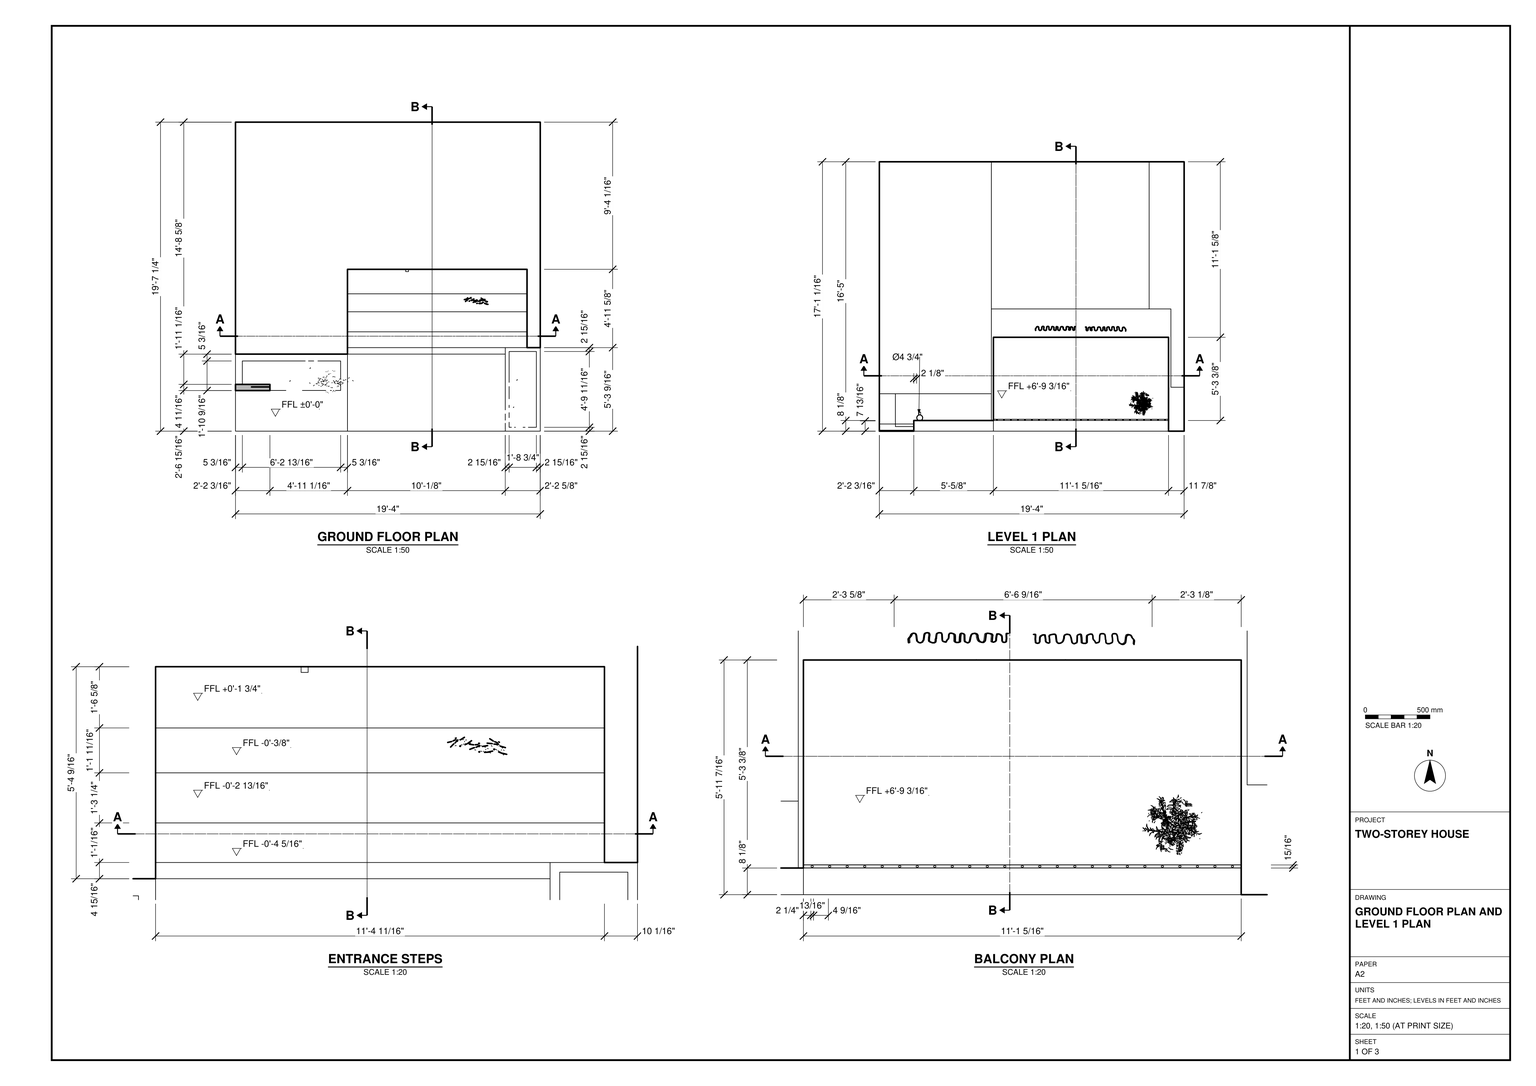
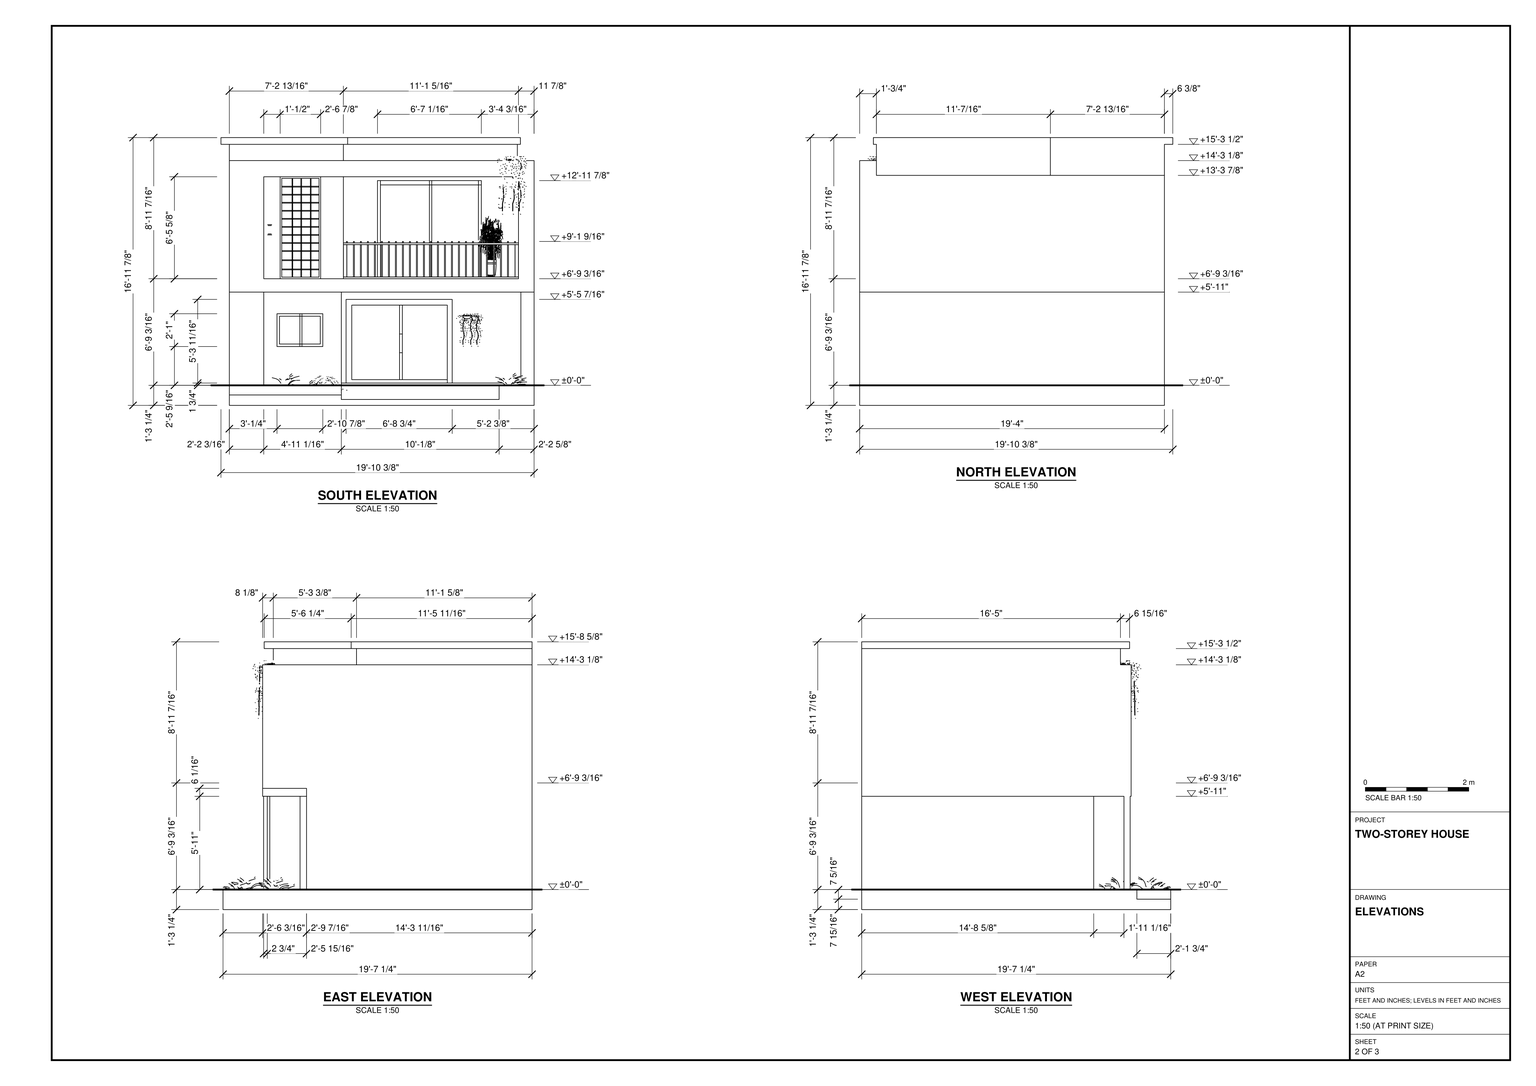
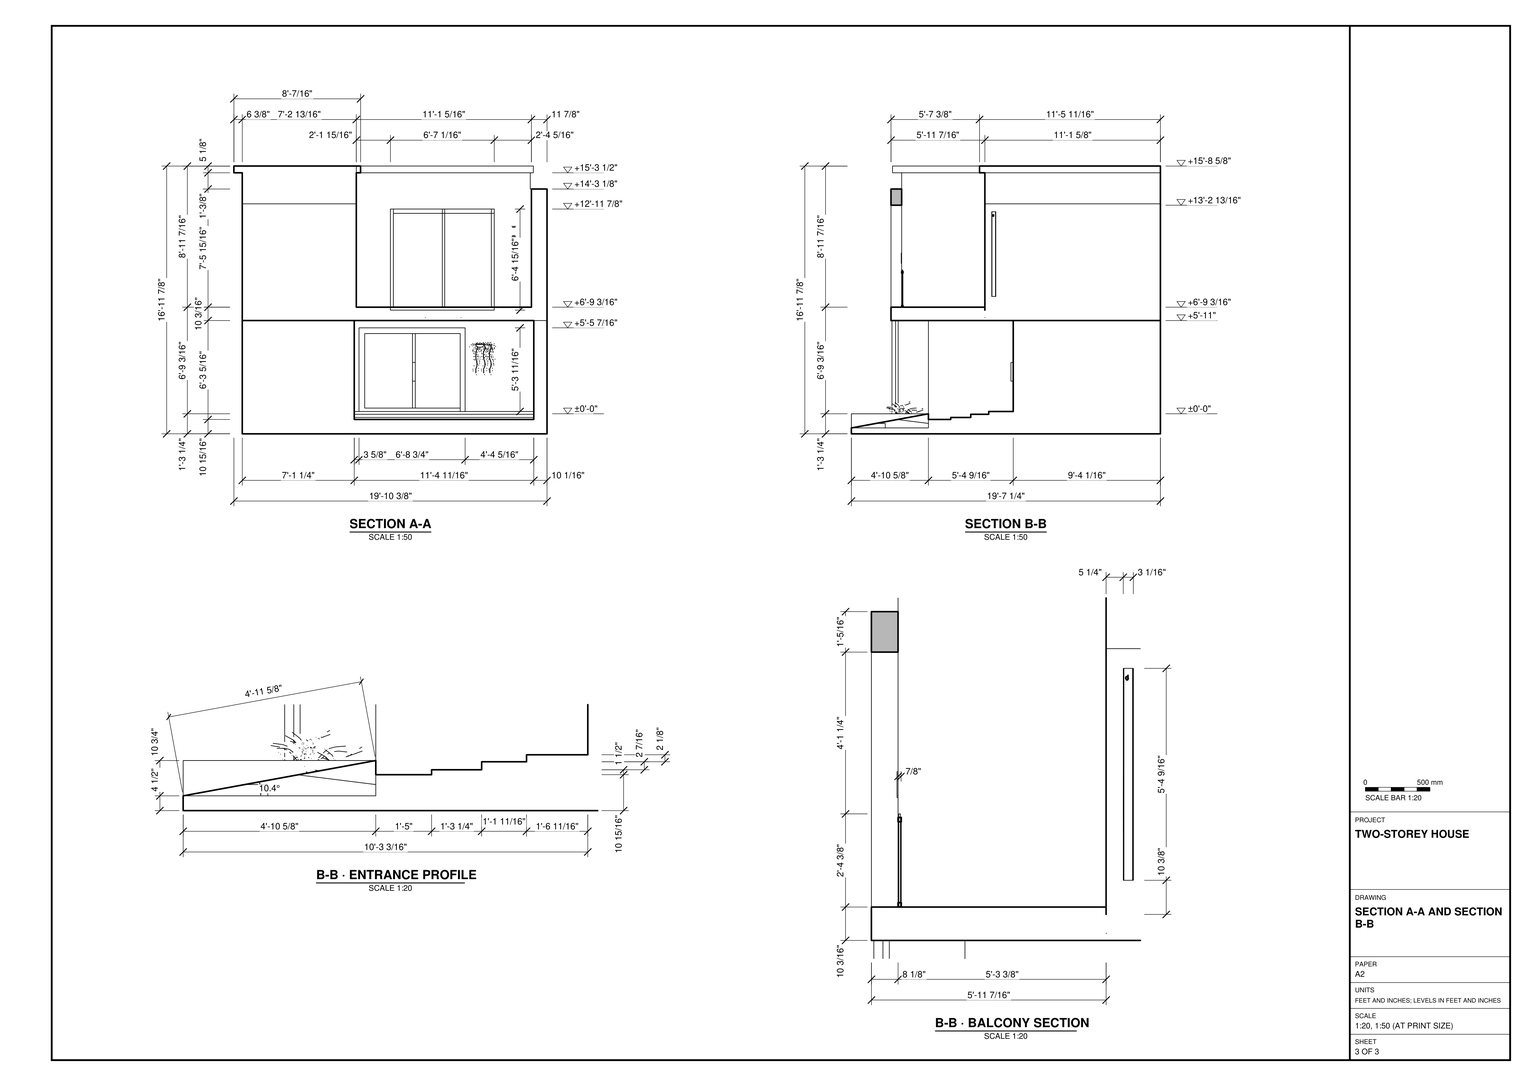
Work in feet and inches to model the two-storey house shown in task_files/diagram_01.pdf. The overall dimensions are 19'-10 3/8" along the south elevation, 19'-7 1/4" from front to back and 16'-11 7/8" high. Set the ground-floor level at ±0'-0" and the upper-floor level at +6'-9 3/16".

Build the base, exterior walls, floor slabs and flat roof with the thicknesses and setbacks shown in the plans and sections. Use the entrance profile on sheet 3 to shape the sloping approach and the shallow steps leading back to the recessed ground-floor entrance. On the south elevation, place the small divided window to the left of the wide glazed entrance. Above it, distinguish the tall gridded opening on the left from the paired glazed opening behind the balcony. Match the balcony footprint to its enlarged plan and place the railing along its outer edge. Include the planting at the entrance and balcony in the positions shown. Decor and loose items, including plants, may be any suitable library components.

Keep the walls, slabs and roof as separate groups or components. Keep each furniture or joinery piece separate and use components for repeated parts. Save one SketchUp model as output_files/two_storey_house_with_a_balcony_and_stepped_entrance.skp.

# SketchUp Ruby script. Lengths in inches.
U = 1.inch
M = Sketchup.active_model
def pt(a) = Geom::Point3d.new(a.map { |v| v * U })
def face(e, loops, mat)
  f = e.add_face(loops[0].map { |a| pt(a) })
  loops[1..].each { |l| e.add_face(l.map { |a| pt(a) }).erase! }
  f.material = f.back_material = mat if mat
  f
end
# faces: each face lists its corners as indices into pts; further lists are holes
def faces(e, pts, list, mat = nil) = list.each { |f| face(e, (f[0].is_a?(Array) ? f : [f]).map { |l| l.map { |i| pts[i] } }, mat) }
# xy, xz, yz: faces in a plane at the given z, y or x. An outline is a flat list of corners, or four numbers for a rectangle; further outlines are holes
def ring(l) = l.size == 4 ? [[l[0], l[1]], [l[2], l[1]], [l[2], l[3]], [l[0], l[3]]] : l.each_slice(2).to_a
def flat(e, list, mat, &to3) = list.each { |f| face(e, (f[0].is_a?(Array) ? f : [f]).map { |l| ring(l).map { |u, v| to3.(u, v) } }, mat) }
def xy(e, z, list, mat = nil) = flat(e, list, mat) { |x, y| [x, y, z] }
def xz(e, y, list, mat = nil) = flat(e, list, mat) { |x, z| [x, y, z] }
def yz(e, x, list, mat = nil) = flat(e, list, mat) { |y, z| [x, y, z] }
def lines(e, pts, list) = list.each { |a, b| e.add_line(pt(pts[a]), pt(pts[b])) }
# prism: a flat outline (further loops are holes) pulled along v
def prism(e, loops, v, mat = nil)
  f = face(e, loops, mat); d = Geom::Vector3d.new(v.map { |x| x * U })
  f.pushpull(f.normal.samedirection?(d) ? d.length : -d.length)
end
def box(e, o, s, mat = nil) = prism(e, [[o, [o[0] + s[0], o[1], o[2]], [o[0] + s[0], o[1] + s[1], o[2]], [o[0], o[1] + s[1], o[2]]]], [0, 0, s[2]], mat)
def at(x, y, z, deg = 0) = Geom::Transformation.translation(pt([x, y, z])) * Geom::Transformation.rotation(ORIGIN, Z_AXIS, deg.degrees)
def axes(o, x, y, z) = Geom::Transformation.new([*x, 0, *y, 0, *z, 0, *pt(o).to_a, 1])
def part(name) = M.definitions.add(name)
# library, detail: a bought-in or finely detailed component or shape, given as its bounding box
def library(name, o, s) = part(name).tap { |d| box(d.entities, o, s) }
def detail(e, o, s) = box(e.add_group.entities, o, s)
def put(e, d, t, mat = nil) = e.add_instance(d, t).tap { |i| i.material = mat if mat }
def group(e, t, mat = nil) = e.add_group.tap { |g| g.transformation = t; g.material = mat if mat }.entities
root = M.entities
M.materials.add("Leaf_Half_Top_007").color = [114, 127, 96]
M.materials.add("Niraj_Hair_Gray").color = [178, 178, 178]
M.materials.add("[Asphalt New]").color = [67, 60, 62]
M.materials.add("[Asphalt_New]").color = [58, 58, 58]
M.materials.add("[Color M08]").color = [30, 30, 30]
M.materials.add("[Color_F18]").color = [71, 102, 40]
M.materials.add("[Groundcover_Wood_Mix]").color = [22, 20, 19]
M.materials.add("[Metal Seamed]").color = [118, 119, 115]
M.materials.add("[Translucent Glass Gray]").color = [128, 128, 128]
M.materials["[Translucent Glass Gray]"].alpha = 0.5
M.materials.add("[Wood Board Cork]").color = [215, 201, 115]
c1 = part("Group\#428")
prism(c1.entities,[[[0,1.97,0],[0,1.97,1.18],[0,0,1.18],[0,0,0]],[[0,1.92,1.13],[0,1.92,0.05],[0,0.05,0.05],[0,0.05,1.13]]],[98.43,0,0])
c2 = part("Group\#430")
xy(c2.entities,0,[[0.3,0,0.22,0.01,0.15,0.04,0.09,0.09,0.04,0.15,0.01,0.22,0,0.3,0.3,0.3],[0.3,0,0.3,0.3,0.59,0.3,0.58,0.22,0.55,0.15,0.5,0.09,0.44,0.04,0.37,0.01],[0,0.3,0.01,0.37,0.04,0.44,0.09,0.5,0.15,0.55,0.22,0.58,0.3,0.59,0.3,0.3],[0.3,0.3,0.3,0.59,0.37,0.58,0.44,0.55,0.5,0.5,0.55,0.44,0.58,0.37,0.59,0.3]])
xy(c2.entities,39.37,[[0.3,0,0.37,0.01,0.44,0.04,0.5,0.09,0.55,0.15,0.58,0.22,0.59,0.3,0.58,0.37,0.55,0.44,0.5,0.5,0.44,0.55,0.37,0.58,0.3,0.59,0.22,0.58,0.15,0.55,0.09,0.5,0.04,0.44,0.01,0.37,0,0.3,0.01,0.22,0.04,0.15,0.09,0.09,0.15,0.04,0.22,0.01]])
p = [[0.09,0.09,0],[0.15,0.04,0],[0.15,0.04,39.37],[0.09,0.09,39.37],[0.22,0.01,0],[0.22,0.01,39.37],
  [0.3,0,0],[0.3,0,39.37],[0.37,0.01,0],[0.37,0.01,39.37],[0.44,0.04,0],[0.44,0.04,39.37],
  [0.5,0.09,0],[0.5,0.09,39.37],[0.01,0.22,0],[0.04,0.15,0],[0.04,0.15,39.37],[0.01,0.22,39.37],
  [0.55,0.15,0],[0.55,0.15,39.37],[0.58,0.22,0],[0.58,0.22,39.37],[0,0.3,0],[0,0.3,39.37],
  [0.59,0.3,0],[0.59,0.3,39.37],[0.01,0.37,0],[0.01,0.37,39.37],[0.58,0.37,0],[0.58,0.37,39.37],
  [0.09,0.5,0],[0.04,0.44,0],[0.04,0.44,39.37],[0.09,0.5,39.37],[0.55,0.44,0],[0.5,0.5,0],
  [0.5,0.5,39.37],[0.55,0.44,39.37],[0.15,0.55,0],[0.15,0.55,39.37],[0.44,0.55,0],[0.44,0.55,39.37],
  [0.22,0.58,0],[0.22,0.58,39.37],[0.3,0.59,0],[0.3,0.59,39.37],[0.37,0.58,0],[0.37,0.58,39.37]]
faces(c2.entities,p,[[0,1,2,3],[1,4,5,2],[4,6,7,5],[6,8,9,7],[8,10,11,9],[10,12,13,11],[14,15,16,17],[15,0,3,16],
  [12,18,19,13],[18,20,21,19],[22,14,17,23],[20,24,25,21],[26,22,23,27],[24,28,29,25],[30,31,32,33],[31,26,27,32],
  [34,35,36,37],[28,34,37,29],[38,30,33,39],[35,40,41,36],[42,38,39,43],[44,42,43,45],[46,44,45,47],[40,46,47,41]])
c3 = part("Group\#429")
prism(c3.entities,[[[0.01,0.22,35.83],[0,0.3,35.83],[0.01,0.37,35.83],[0.04,0.44,35.83],[0.09,0.5,35.83],[0.15,0.55,35.83],[0.22,0.58,35.83],[0.3,0.59,35.83],[0.37,0.58,35.83],[0.44,0.55,35.83],[0.5,0.5,35.83],[0.55,0.44,35.83],[0.58,0.37,35.83],[0.59,0.3,35.83],[0.58,0.22,35.83],[0.55,0.15,35.83],[0.5,0.09,35.83],[0.44,0.04,35.83],[0.37,0.01,35.83],[0.3,0,35.83],[0.22,0.01,35.83],[0.15,0.04,35.83],[0.09,0.09,35.83],[0.04,0.15,35.83]]],[0,0,3.54])
c4 = part("Metal railing panel")
g1 = group(c4.entities,at(0,0,0))
put(g1,c1,axes([0,0,39.76],[1,0,0],[0,0,-1],[0,1,0]),"[Color M08]")
put(g1,c1,axes([0,0,1.97],[1,0,0],[0,0,-1],[0,1,0]),"[Color M08]")
put(g1,c1,axes([98.43,0,37.8],[0,0,-0.364],[-1,0,0],[0,1,0]),"[Color M08]")
put(g1,c1,axes([1.97,0,37.8],[0,0,-0.364],[-1,0,0],[0,1,0]),"[Color M08]")
g2 = group(c4.entities,at(1.67,0.3,1.97))
put(g2,c2,at(78.74,0,0),"[Color M08]")
put(g2,c2,at(90.55,0,0),"[Color M08]")
put(g2,c2,at(82.68,0,0),"[Color M08]")
put(g2,c2,at(86.61,0,0),"[Color M08]")
put(g2,c2,at(66.93,0,0),"[Color M08]")
put(g2,c2,at(11.8125,0,0),"[Color M08]")
put(g2,c2,at(15.75,0,0),"[Color M08]")
put(g2,c2,at(47.24,0,0),"[Color M08]")
put(g2,c2,at(59.06,0,0),"[Color M08]")
put(g2,c3,at(0,0,0),"[Color M08]")
put(g2,c2,at(39.37,0,0),"[Color M08]")
put(g2,c2,at(62.99,0,0),"[Color M08]")
put(g2,c2,at(55.12,0,0),"[Color M08]")
put(g2,c2,at(19.69,0,0),"[Color M08]")
put(g2,c2,at(35.43,0,0),"[Color M08]")
put(g2,c2,at(7.875,0,0),"[Color M08]")
put(g2,c2,at(23.62,0,0),"[Color M08]")
put(g2,c2,at(31.5,0,0),"[Color M08]")
put(g2,c2,at(43.31,0,0),"[Color M08]")
put(g2,c2,at(27.56,0,0),"[Color M08]")
put(g2,c2,at(3.9375,0,0),"[Color M08]")
put(g2,c2,at(51.18,0,0),"[Color M08]")
put(g2,c2,at(70.87,0,0),"[Color M08]")
put(g2,c2,at(74.8,0,0),"[Color M08]")
put(g2,c3,at(94.49,0,0),"[Color M08]")
c5 = library("Broadleaf plant",[0,0,0],[149.19,166.1,98.1875])
c6 = library("TS_VASO+GANCHOS-PARA-PENDURAR\#1",[-17.61,-15.74,-70.29],[36.55,50.24,77.96])
c7 = part("Pot Half 03")
p = [[1.24,1.853,0],[6.161,1.853,0],[6.586,1.426,3.732],[0.815,1.426,3.732],[1.24,1.851,0],[6.161,7.34,0],
  [6.586,7.767,3.732],[6.679,1.345,4.342],[0.722,1.345,4.342],[6.679,7.848,4.342],[6.772,1.24,4.958],[0.629,1.24,4.958],
  [6.772,7.953,4.958],[6.906,1.118,5.538],[0.495,1.118,5.538],[6.906,8.075,5.538],[7.045,0.967,6.137],[0.356,0.967,6.137],
  [7.045,8.226,6.137],[7.221,0.804,6.691],[0.18,0.804,6.691],[7.221,8.389,6.691],[7.401,0.616,7.25],[0,0.616,7.25],
  [7.401,8.577,7.25]]
faces(c7.entities,p,[[0,1,2,3],[3,0,4],[5,6,2,1],[7,8,3,2],[9,7,2,6],[10,11,8,7],[12,10,7,9],[13,14,11,10],
  [15,13,10,12],[16,17,14,13],[18,16,13,15],[19,20,17,16],[21,19,16,18],[22,23,20,19],[24,22,19,21]],"[Asphalt_New]")
c8 = part("Dirt 003")
xy(c8.entities,-0.75,[[0,-3.72,3.43,-3.72,3.43,0],[-3.43,0,0,3.72,-3.43,3.72]])
p = [[-3.43,-3.72,-0.75],[0,0,0],[-3.43,0,-0.75],[0,-3.72,-0.75],[3.43,0,-0.75],[0,3.72,-0.75],
  [3.43,3.72,-0.75]]
faces(c8.entities,p,[[0,1,2],[0,3,1],[3,4,1],[2,1,5],[1,4,6],[1,6,5]])
c9 = part("Planter Box 01")
put(c9.entities,c7,axes([-30.22,-0.62,-6.86],[4.97512,0,0],[0,1,0],[0,0,1]),"[Asphalt_New]")
put(c9.entities,c7,axes([6.66,8.58,-6.86],[-4.97512,0,0],[0,-1,0],[0,0,1]))
put(c9.entities,c8,axes([-11.66,3.97,0.41],[4.97512,0,0],[0,1,0],[0,0,1]),"[Groundcover_Wood_Mix]")
c10 = part("Group8\#1")
p = [[88.35,32.45,7.18],[88.36,32.39,7.24],[86.45,32.02,7.22],[86.4375,32.08,7.17],[88.36,32.39,7.32],[86.45,32.02,7.3],
  [88.33,32.52,7.2],[86.42,32.16,7.1875],[88.32,32.56,7.28],[86.42,32.19,7.26],[90.24,33.16,7.22],[90.27,33.09,7.2],
  [90.29,33.02,7.26],[90.29,33.02,7.34],[90.23,33.19,7.3],[88.34,32.45,7.37],[86.4375,32.08,7.35],[88.32,32.52,7.35],
  [86.42,32.16,7.34],[90.27,33.08,7.39],[90.24,33.16,7.37]]
faces(c10.entities,p,[[0,1,2,3],[1,4,5,2],[6,0,3,7],[8,6,7,9],[10,11,0,6],[11,12,1,0],[12,13,4,1],[14,10,6,8],
  [4,15,16,5],[15,17,18,16],[17,8,9,18],[13,19,15,4],[19,20,17,15],[20,14,8,17]],"[Color_F18]")
c11 = part("Stem Segment 03")
put(c11.entities,c10,at(-88.34,-32.47,-7.28))
c12 = part("Leaf Stem 003")
p = [[2.85,0.02,0.06],[2.46,0.65,0.09],[2.46,0.65,0.03],[2.85,0.02,0.02],[2.92,0.03,0.01],[2.53,0.71,0.01],
  [2.55,0.72,0.0625],[2.93,0.04,0.04],[2.49,0.68,0],[2.89,0.01,0],[2.92,0.03,0.07],[2.53,0.71,0.11],
  [1.77,1.25,0.09],[1.77,1.25,0.03],[2.46,0.65,0.09],[1.8,1.29,0],[1.83,1.33,0.01],[1.84,1.35,0.0625],
  [1.38,1.49,0.09],[1.38,1.49,0.03],[1.43,1.57,0.01],[1.44,1.59,0.0625],[1.4,1.52,0],[0.375,2.11,0.09],
  [0.375,2.11,0.03],[0.39,2.15,0],[0.42,2.19,0.01],[0.43,2.22,0.0625],[0,2.29,0.05],[0.02,2.35,0],
  [0,2.29,0.13],[0,2.29,0.09],[0.04,2.43,0.02],[0.06,2.46,0.09],[2.49,0.68,0.12],[2.89,0.01,0.08],
  [1.83,1.33,0.11],[1.8,1.29,0.12],[1.4,1.52,0.12],[1.43,1.57,0.11],[0.42,2.19,0.11],[0.39,2.15,0.12],
  [0.02,2.35,0.1875],[0.04,2.43,0.17]]
faces(c12.entities,p,[[0,1,2,3],[4,5,6,7],[8,5,4,9],[10,7,6,11],[9,3,2,8],[12,13,2,14],[2,13,8],[15,8,13],
  [8,15,5],[16,5,15],[17,6,16],[5,16,6],[13,12,18,19],[17,16,20,21],[16,15,22,20],[15,13,19,22],
  [19,18,23,24],[22,19,24,25],[20,22,25,26],[21,20,26,27],[24,28,25],[29,25,28],[25,29,26],[30,31,28,24,23],
  [32,26,29],[33,27,32],[26,32,27],[34,35,10,11],[11,6,36],[17,36,6],[34,11,37],[36,37,11],
  [37,12,34],[14,34,12],[12,37,38,18],[37,36,39,38],[36,17,21,39],[38,39,40,41],[18,38,41,23],[39,21,27,40],
  [41,40,42],[30,23,41,42],[43,42,40],[40,27,43],[33,43,27]],"[Color_F18]")
c13 = part("Leaf stalk")
put(c13.entities,c12,at(0,0,0),"[Color_F18]")
c14 = part("Leaf Half 003\#2")
xz(c14.entities,0,[[5.394,0.387,3.719,3.029,4.031,3.19,4.352,3.332,4.681,3.455,5.017,3.558,5.359,3.64,5.704,3.702,6.053,3.743,6.404,3.763,6.755,3.762,6.968,3.765,7.18,3.761,7.392,3.75,7.604,3.731,7.815,3.706,8.025,3.674,8.234,3.635,8.442,3.589,8.648,3.537,8.852,3.478,9.054,3.412,9.254,3.339,9.523,3.226,9.776,3.081,10.009,2.905,10.218,2.701,10.4,2.473,10.553,2.224,10.674,1.959,10.76,1.68,10.803,1.439,10.807,1.344,10.806,1.249,10.8,1.154,10.788,1.059,10.772,0.965,10.749,0.873,10.722,0.781,10.689,0.69,10.652,0.602,10.609,0.515,10.562,0.43,10.535,0.387]],"Leaf_Half_Top_007")
p = [[0.878,-0.545,0.444],[0.896,-0.538,0.464],[0.931,-0.525,0.507],[0.966,-0.512,0.549],[1.39,-0.366,0.995],[1.791,-0.364,0.444],
  [2.095,-0.165,1.727],[1.842,-0.358,0.429],[1.796,-0.364,0.437],[2.997,-0.164,0.429],[2.858,-0.042,2.43],[3.012,-0.163,0.428],
  [4.203,-0.043,0.406],[2.861,-0.041,2.432],[3.719,0,3.029],[5.394,0,0.387],[2.302,-0.122,1.934],[2.485,-0.09,2.102],
  [2.671,-0.064,2.268],[3.132,-0.018,2.649],[3.418,-0.005,2.848]]
faces(c14.entities,p,[[0,1,2,3,4,5],[5,4,6,7,8],[7,6,9],[9,6,10,11],[11,10,12],[10,13,14,12],[15,12,14],[16,10,6],
  [17,10,16],[18,10,17],[19,14,13],[20,14,19]],"Leaf_Half_Top_007")
c15 = part("Leaf  003")
put(c15.entities,c14,axes([0.38,-0.76,0.25],[-0.73627,0.51406,-0.06038],[0.07956,0.22794,0.97042],[-0.56957,-0.78855,0.23191]))
put(c15.entities,c14,axes([-0.33,-1.74,0.14],[-0.71206,0.54726,-0.05889],[-0.2936,-0.28379,0.91283],[0.5365,0.74143,0.40305]))
c16 = part("Stem 03")
put(c16.entities,c11,axes([-3.94,-0.51,0],[1.00831,0.3173,0.48929],[0.62823,-0.33003,-1.08062],[-0.15419,1.18746,-0.4523]))
put(c16.entities,c11,axes([3.49,-0.02,-2.22],[0.59576,-0.02646,-0.80273],[0.76313,-0.29296,0.57602],[-0.25041,-0.95576,-0.15434]))
put(c16.entities,c11,axes([9.375,1.32,-6.76],[0.76506,0.42795,-0.48118],[0.54249,-0.02572,0.83967],[0.34696,-0.90343,-0.25184]))
put(c16.entities,c11,axes([6.35,0.02,-4.79],[0.59576,-0.02646,-0.80273],[0.35669,0.9042,0.23492],[0.71961,-0.42629,0.54812]))
put(c16.entities,c11,axes([12.62,2.51,-7.16],[0.6803,0.33788,-0.02508],[0.33232,-0.6545,0.19696],[0.06597,-0.18727,-0.73361]),"[Color_F18]")
put(c16.entities,c11,axes([0.3,0.04,-0.21],[-0.84454,-0.08139,0.52927],[-0.53545,0.11632,-0.83652],[0.00652,-0.98987,-0.14182]))
put(c16.entities,c13,axes([-1.3125,-1.96,2.02],[0.30666,0.85318,0.66121],[-0.04993,0.77839,-0.74104],[-2.0519,0.10857,0.11685]))
put(c16.entities,c13,axes([-4.65,-2.32,1.92],[0.24338,0.85318,0.71076],[0.37608,0.73871,-0.80238],[-1.59205,0.25393,-0.07463]))
put(c16.entities,c13,axes([-7.2,-3.29,1.22],[0.30238,0.83595,0.58629],[0.37608,0.73871,-0.65859],[-1.58433,0.30016,-0.01484]))
put(c16.entities,c13,axes([0.53,-1.96,0.51],[0.32572,0.6177,0.78674],[-0.09946,0.84405,-0.28154],[-1.60731,-0.00658,0.27494]))
put(c16.entities,c13,axes([3.92,-1.49,-0.93],[0.30617,0.58064,0.73954],[-0.72502,0.69723,-0.01619],[-1.09889,-0.4139,0.62826]))
put(c16.entities,c13,axes([4.9375,-1.13,-0.64],[0.15705,0.93505,0.23221],[-0.515,0.47073,-0.69124],[-1.33185,0.0406,0.34107]))
put(c16.entities,c13,axes([6.62,-2.02,-3.44],[0.25326,0.61577,0.6588],[-0.59973,0.73941,-0.01442],[-0.90899,-0.43895,0.55966]))
put(c16.entities,c13,axes([7.8,1.95,-4.46],[0.47026,-0.74247,0.15265],[-0.05932,-0.60353,-0.69183],[0.55983,0.33909,-0.83034]))
put(c16.entities,c13,axes([8.1,0.54,-5.54],[0.44324,0.59809,0.36462],[0.53568,0.30234,-0.47352],[-0.95326,0.41061,-0.31748]))
put(c16.entities,c13,axes([9.91,3.23,-5.95],[0.66281,-0.36564,0.35664],[0.55741,-0.47264,-0.48381],[0.53295,0.52862,-0.61482]))
put(c16.entities,c13,axes([13.4375,2.48,-5.88],[0.62226,-0.02903,-0.01582],[0.2868,0.07076,-0.50026],[-0.12016,0.85017,-0.2373]))
put(c16.entities,c15,axes([14.48,0.92,-5.23],[0.0087,-0.21722,0.04751],[0.21837,-0.00716,-0.09125],[0.14863,0.04515,0.19139]))
put(c16.entities,c15,axes([9.9,3.39,-4.35],[-0.29123,0.01957,0.06847],[-0.02535,-0.26587,-0.00841],[0.07568,-0.01372,0.26066]))
put(c16.entities,c15,axes([7.01,1.24,-3.35],[-0.21895,-0.20956,0.10962],[0.2232,-0.10618,-0.07961],[0.2062,0.0234,0.22464]))
put(c16.entities,c15,axes([9.1,-1.16,-2.97],[0.16646,-0.16408,0.06345],[0.32123,-0.02918,-0.16141],[0.19487,0.1494,0.19131]))
put(c16.entities,c15,axes([7.62,1.91,-0.74],[-0.13636,0.15771,0.21131],[-0.30082,-0.24908,0.19555],[0.22388,-0.05253,0.25505]))
put(c16.entities,c15,axes([6.63,0.34,1.27],[0.28289,-0.14866,0.08879],[0.17621,0.08243,-0.1563],[0.15509,0.20742,0.13835]))
put(c16.entities,c15,axes([5.87,-2.37,2.55],[0.24481,-0.24553,0.03382],[0.13933,0.2091,-0.24174],[0.19372,0.29074,0.28289]))
put(c16.entities,c15,axes([2.0625,1.79,5.35],[-0.18104,0.18123,0.28972],[-0.43052,-0.16317,-0.07437],[0.10324,-0.22668,0.29612]))
put(c16.entities,c15,axes([1.29,-0.99,6.37],[0.35078,-0.04064,0.25637],[0.22081,0.3154,-0.13622],[-0.24663,0.21043,0.25293]))
put(c16.entities,c13,axes([-3.94,-4.26,-2.18],[0.2039,-0.7121,1.03293],[-0.70199,1.01563,0.56503],[-1.36054,-0.65537,-0.37049]))
c17 = part("3D Plant 003")
put(c17.entities,c9,axes([2.34,-3.97,-0.41],[0.201,0,0],[0,1,0],[0,0,1]))
put(c17.entities,c16,axes([5.43,0.67,0.04],[0.90233,-0.11399,0],[0.12659,1.00204,0],[0,0,1]))
put(c17.entities,c16,axes([4.56,-0.51,-0.05],[0.64048,0.07982,0.02703],[0.12375,-0.99231,-0.00197],[-0.04128,-0.00713,0.99912]))
put(c17.entities,c16,axes([-4.94,1.31,0.19],[-0.72845,-0.05489,0.02686],[-0.09535,1.18483,-0.16456],[0.02598,0.13957,0.98987]))
put(c17.entities,c16,axes([-5.64,-0.91,0.07],[-0.88284,0.04315,-0.01389],[-0.04884,-0.99881,0.00119],[-0.01547,0.00194,0.98988]))
put(c17.entities,c16,axes([3.75,-0.16,0.2],[0.377,-0.2222,0.04965],[0.26332,0.45308,0.02828],[-0.07969,0.00668,0.63498]))
put(c17.entities,c16,axes([-3.77,0.34,0.13],[-0.41282,0.07246,0.03267],[-0.09028,-0.51695,0.00573],[0.05019,-0.00169,0.63803]))
put(c17.entities,c16,axes([-3.89,-2.29,0.13],[-0.43617,-0.01963,0.05782],[0.02879,-0.5225,0.03978],[0.0815,0.05265,0.6326]))
put(c17.entities,c16,axes([3.46,-1.51,0.15],[0.34649,-0.00968,0.11609],[-0.02228,-0.52383,0.02283],[-0.16372,0.02836,0.49105]))
put(c17.entities,c15,axes([-3.23,-10.97,0.92],[0.14719,-0.61301,-0.08966],[0.60937,0.12663,0.13459],[-0.11174,-0.11691,0.6159]))
put(c17.entities,c15,axes([3.22,-9.64,-1.72],[0.47123,-0.37571,-0.20559],[0.42416,0.3671,0.30134],[-0.05927,-0.35994,0.52193]))
put(c17.entities,c15,axes([0.79,-6.4375,1.4375],[0.21976,-0.38322,0.22587],[0.34942,0.30462,0.17686],[-0.27528,0.08073,0.40481]))
put(c17.entities,c15,axes([1.99,4.79,6.88],[-0.22806,0.40163,0.2359],[-0.48816,-0.16923,-0.16491],[-0.06681,-0.43854,0.27612]))
put(c17.entities,c15,axes([-5.22,3.625,7.43],[-0.47836,-0.1205,0.2836],[-0.03228,-0.53536,-0.2994],[0.3042,-0.26534,0.41616]))
put(c17.entities,c15,axes([-2.24,-5.2,5.32],[0.19023,-0.33022,0.3177],[0.44902,0.20297,-0.05789],[-0.09143,0.30972,0.37668]))
put(c17.entities,c15,axes([3.33,-0.44,5.29],[0.46715,-0.167,0.15853],[-0.081,-0.39547,-0.27311],[-0.27014,-0.20951,0.34065]))
put(c17.entities,c15,axes([6.9,-4.43,-0.17],[0.51342,-0.02023,0.07039],[-0.0428,0.28715,0.45809],[-0.24354,-0.33353,0.32011]))
put(c17.entities,c15,axes([-6.28,-3.56,1.22],[-0.63664,-0.02023,0.07039],[0.05307,0.28715,0.45809],[0.30199,-0.33353,0.32011]))
put(c17.entities,c15,axes([0.92,-0.57,3.76],[-0.19279,0.26754,0.24313],[-0.36734,-0.21658,-0.04151],[0.07959,-0.3505,0.20299]))
put(c17.entities,c15,axes([-3.42,9.06,-2.66],[0.1891,0.43607,-0.42375],[0.60746,-0.11599,0.15173],[-0.02672,0.44931,0.45044]))
put(c17.entities,c15,axes([2.95,9.4,-1.4375],[0.42849,0.29992,-0.18263],[0.40356,-0.42673,0.24603],[0.00748,0.32333,0.54853]))
put(c17.entities,c15,axes([-2.67,6.99,2.51],[-0.57491,0.28187,-0.02654],[-0.2288,-0.49271,0.00048],[0.15861,-0.20895,0.48589]))
c18 = library("CURTAIN\#1",[-0.6,-7.68,-83.58],[11.58,83.5,83.58])
c19 = library("Wall+Light",[81.37,10.74,0],[4.72,6.69,7.875])
c20 = library("Group\#173",[-2.88,-2.59,0],[25.32,25.32,25.27])
xy(root,0,[[6.375,0,238.375,235.25]])
xy(root,8.125,[[214.69,2.94,235.43,60.65]])
xy(root,8.5625,[[11.58,30.99,16.44,30.99,16.44,35.61,32.59,35.61,32.59,30.99,86.42,30.99,86.42,53.44,11.58,53.44]])
xy(root,10.9375,[[91.625,58.65,211.75,63.59],[91.625,63.59,228.31,75.64]])
xy(root,12.4375,[[91.625,75.64,228.31,90.89]])
xy(root,14.875,[[91.625,90.89,228.31,104.5625]])
xy(root,15.25,[[6.375,0,91.625,0,91.625,58.65,6.375,58.65,6.375,35.61,11.58,35.61,11.58,53.44,86.42,53.44,86.42,30.99,32.59,30.99,32.59,30.91,6.375,30.91],[[211.75,0,238.375,63.59],[214.69,2.94,235.43,60.65]],[6.375,30.91,11.58,33.67],[11.58,30.91,16.44,30.99],[16.44,30.91,32.59,33.67],
  [11.58,30.99,16.44,33.67],[6.375,33.67,11.58,35.61],[11.58,33.67,16.44,35.61],[16.44,33.67,32.59,35.61]])
xy(root,17,[[91.625,104.5625,228.31,123.22]])
xy(root,40.11,[[135.94,121.47,138.08,123.22]],"[Metal Seamed]")
xy(root,54.35,[[135.94,121.47,138.08,123.22]],"[Metal Seamed]")
xy(root,86.25,[[6.375,30.16,32.59,30.91],[32.59,30.16,91.625,30.91],[91.625,30.16,91.625,123.22,228.31,123.22,228.31,63.59,238.375,63.59,238.375,30.16],[6.375,35.61,18.56,58.65],[6.375,58.65,91.625,235.25],
  [91.625,123.22,211.75,235.25]])
xy(root,86.29,[[18.56,33.67,32.59,35.61]])
xy(root,96.42,[[32.59,30.16,93.19,38.28],[93.19,30.16,226.5,101.625]])
xy(root,172.75,[[225.62,30.16,226.5,30.91]])
xy(root,174.06,[[[32.59,30.16,32.59,38.28,225.625,38.28,225.63,30.91,225.62,30.91,225.62,30.16],[124.72,33.26,125.24,33.33,125.72,33.53,126.13,33.85,126.45,34.26,126.65,34.74,126.72,35.26,126.65,35.78,126.45,36.26,126.13,36.67,125.72,36.99,125.24,37.19,124.72,37.26,124.2,37.19,123.72,36.99,123.3,36.67,122.99,36.26,122.79,35.78,122.72,35.26,122.79,34.74,122.99,34.26,123.3,33.85,123.72,33.53,124.2,33.33],[81.34,33.26,81.86,33.33,82.34,33.53,82.76,33.85,83.08,34.26,83.28,34.74,83.34,35.26,83.28,35.78,83.08,36.26,82.76,36.67,82.34,36.99,81.86,37.19,81.34,37.26,80.83,37.19,80.34,36.99,79.93,36.67,79.61,36.26,79.41,35.78,79.34,35.26,79.41,34.74,79.61,34.26,79.93,33.85,80.34,33.53,80.83,33.33],[173.72,33.26,174.24,33.33,174.72,33.53,175.13,33.85,175.45,34.26,175.65,34.74,175.72,35.26,175.65,35.78,175.45,36.26,175.13,36.67,174.72,36.99,174.24,37.19,173.72,37.26,173.2,37.19,172.72,36.99,172.3,36.67,171.99,36.26,171.79,35.78,171.72,35.26,171.79,34.74,171.99,34.26,172.3,33.85,172.72,33.53,173.2,33.33]],[225.63,30.91,225.625,38.28,225.63,38.28]])
xy(root,174.06,[[81.34,33.26,80.83,33.33,80.34,33.53,79.93,33.85,79.61,34.26,79.41,34.74,79.34,35.26,79.41,35.78,79.61,36.26,79.93,36.67,80.34,36.99,80.83,37.19,81.34,37.26,81.86,37.19,82.34,36.99,82.76,36.67,83.08,36.26,83.28,35.78,83.34,35.26,83.28,34.74,83.08,34.26,82.76,33.85,82.34,33.53,81.86,33.33],[124.72,33.26,124.2,33.33,123.72,33.53,123.3,33.85,122.99,34.26,122.79,34.74,122.72,35.26,122.79,35.78,122.99,36.26,123.3,36.67,123.72,36.99,124.2,37.19,124.72,37.26,125.24,37.19,125.72,36.99,126.13,36.67,126.45,36.26,126.65,35.78,126.72,35.26,126.65,34.74,126.45,34.26,126.13,33.85,125.72,33.53,125.24,33.33],[173.72,33.26,173.2,33.33,172.72,33.53,172.3,33.85,171.99,34.26,171.79,34.74,171.72,35.26,171.79,35.78,171.99,36.26,172.3,36.67,172.72,36.99,173.2,37.19,173.72,37.26,174.24,37.19,174.72,36.99,175.13,36.67,175.45,36.26,175.65,35.78,175.72,35.26,175.65,34.74,175.45,34.26,175.13,33.85,174.72,33.53,174.24,33.33]],"[Wood Board Cork]")
xy(root,186.375,[[6.375,30.16,238.375,30.16,238.375,235.25,225.62,235.25,225.62,101.625,226.5,101.625,226.5,38.28,6.375,38.28]])
xy(root,198.73,[[0,31.34,16.44,38.28],[16.44,31.34,93.19,38.28],[93.19,31.34,96.44,41.03],[0,38.28,6.375,41.03],[0,41.03,6.375,235.25],
  [93.19,41.03,96.44,101.625],[96.44,97.5625,227.94,101.625],[225.62,101.625,227.94,235.25]])
xy(root,203.875,[[0,31.34,96.44,31.34,96.44,97.5625,227.94,97.5625,227.94,235.25,0,235.25]])
xz(root,0,[[6.375,0,238.375,0,238.375,15.25,211.75,15.25,211.75,4.5,91.625,4.5,91.625,7.9375,6.375,7.9375],[6.375,7.9375,91.625,15.25]])
xz(root,2.94,[[214.69,8.125,235.43,15.25]])
xz(root,30.16,[[[6.375,86.25,238.375,186.375],[32.59,96.42,32.59,174.06,225.62,174.06,225.62,172.75,226.5,172.75,226.5,96.42]]])
xz(root,30.91,[[6.375,15.25,32.59,86.25]])
xz(root,30.99,[[11.58,8.5625,16.44,15.25],[32.59,8.5625,86.42,15.25]])
xz(root,31.34,[[0,198.73,96.44,203.875]])
xz(root,33.67,[[18.56,15.25,32.59,86.29]])
xz(root,35.61,[[16.44,8.5625,32.59,15.25],[6.375,15.25,6.375,86.25,18.56,86.25,18.56,86.29,32.59,86.29,32.59,15.25]])
xz(root,38.28,[[93.19,174.06,225.63,186.375]])
xz(root,38.28,[[32.59,96.42,45.06,174.06],[75.9,96.42,93.19,174.06],[6.375,186.375,93.19,198.73]],"Niraj_Hair_Gray")
xz(root,38.28,[[[45.06,96.42,75.9,174.06],[46.28,97.64,74.68,172.83]],[54.12,97.64,54.63,103.21],[60.8,97.64,61.42,103.21],[68.05,97.64,68.61,103.21],[46.28,103.21,54.12,103.82],
  [54.12,103.21,54.63,103.82],[54.63,103.21,60.8,103.82],[60.8,103.21,61.42,103.82],[61.42,103.21,68.05,103.82],[68.05,103.21,68.61,103.82],
  [68.61,103.21,74.68,103.82],[54.12,103.82,54.63,110.21],[60.8,103.82,61.42,110.21],[68.05,103.82,68.61,110.21],[46.28,110.21,54.12,110.82],
  [54.12,110.21,54.63,110.82],[54.63,110.21,60.8,110.82],[60.8,110.21,61.42,110.82],[61.42,110.21,68.05,110.82],[68.05,110.21,68.61,110.82],
  [68.61,110.21,74.68,110.82],[54.12,110.82,54.63,117.21],[60.8,110.82,61.42,117.21],[68.05,110.82,68.61,117.21],[46.28,117.21,54.12,117.82],
  [54.12,117.21,54.63,117.82],[54.63,117.21,60.8,117.82],[60.8,117.21,61.42,117.82],[61.42,117.21,68.05,117.82],[68.05,117.21,68.61,117.82],
  [68.61,117.21,74.68,117.82],[54.12,117.82,54.63,123.33],[60.8,117.82,61.42,123.33],[68.05,117.82,68.61,123.33],[46.28,123.33,54.12,123.94],
  [54.12,123.33,54.63,123.94],[54.63,123.33,60.8,123.94],[60.8,123.33,61.42,123.94],[61.42,123.33,68.05,123.94],[68.05,123.33,68.61,123.94],
  [68.61,123.33,74.68,123.94],[54.12,123.94,54.63,129.46],[60.8,123.94,61.42,129.46],[68.05,123.94,68.61,129.46],[46.28,129.46,54.12,130.07],
  [54.12,129.46,54.63,130.07],[54.63,129.46,60.8,130.07],[60.8,129.46,61.42,130.07],[61.42,129.46,68.05,130.07],[68.05,129.46,68.61,130.07],
  [68.61,129.46,74.68,130.07],[54.12,130.07,54.63,135.58],[60.8,130.07,61.42,135.58],[68.05,130.07,68.61,135.58],[46.28,135.58,54.12,136.19],
  [54.12,135.58,54.63,136.19],[54.63,135.58,60.8,136.19],[60.8,135.58,61.42,136.19],[61.42,135.58,68.05,136.19],[68.05,135.58,68.61,136.19],
  [68.61,135.58,74.68,136.19],[54.12,136.19,54.63,141.71],[60.8,136.19,61.42,141.71],[68.05,136.19,68.61,141.71],[46.28,141.71,54.12,142.32],
  [54.12,141.71,54.63,142.32],[54.63,141.71,60.8,142.32],[60.8,141.71,61.42,142.32],[61.42,141.71,68.05,142.32],[68.05,141.71,68.61,142.32],
  [68.61,141.71,74.68,142.32],[54.12,142.32,54.63,147.83],[60.8,142.32,61.42,147.83],[68.05,142.32,68.61,147.83],[46.28,147.83,54.12,148.44],
  [54.12,147.83,54.63,148.44],[54.63,147.83,60.8,148.44],[60.8,147.83,61.42,148.44],[61.42,147.83,68.05,148.44],[68.05,147.83,68.61,148.44],
  [68.61,147.83,74.68,148.44],[54.12,148.44,54.63,153.96],[60.8,148.44,61.42,153.96],[68.05,148.44,68.61,153.96],[46.28,153.96,54.12,154.57],
  [54.12,153.96,54.63,154.57],[54.63,153.96,60.8,154.57],[60.8,153.96,61.42,154.57],[61.42,153.96,68.05,154.57],[68.05,153.96,68.61,154.57],
  [68.61,153.96,74.68,154.57],[54.12,154.57,54.63,160.08],[60.8,154.57,61.42,160.08],[68.05,154.57,68.61,160.08],[46.28,160.08,54.12,160.69],
  [54.12,160.08,54.63,160.69],[54.63,160.08,60.8,160.69],[60.8,160.08,61.42,160.69],[61.42,160.08,68.05,160.69],[68.05,160.08,68.61,160.69],
  [68.61,160.08,74.68,160.69],[54.12,160.69,54.63,166.21],[60.8,160.69,61.42,166.21],[68.05,160.69,68.61,166.21],[46.28,166.21,54.12,166.82],
  [54.12,166.21,54.63,166.82],[54.63,166.21,60.8,166.82],[60.8,166.21,61.42,166.82],[61.42,166.21,68.05,166.82],[68.05,166.21,68.61,166.82],
  [68.61,166.21,74.68,166.82],[54.12,166.82,54.63,172.83],[60.8,166.82,61.42,172.83],[68.05,166.82,68.61,172.83]],"[Asphalt New]")
xz(root,38.28,[[46.28,97.64,54.12,103.21],[54.63,97.64,60.8,103.21],[61.42,97.64,68.05,103.21],[68.61,97.64,74.68,103.21],[46.28,103.82,54.12,110.21],
  [54.63,103.82,60.8,110.21],[61.42,103.82,68.05,110.21],[68.61,103.82,74.68,110.21],[46.28,110.82,54.12,117.21],[54.63,110.82,60.8,117.21],
  [61.42,110.82,68.05,117.21],[68.61,110.82,74.68,117.21],[46.28,117.82,54.12,123.33],[54.63,117.82,60.8,123.33],[61.42,117.82,68.05,123.33],
  [68.61,117.82,74.68,123.33],[46.28,123.94,54.12,129.46],[54.63,123.94,60.8,129.46],[61.42,123.94,68.05,129.46],[68.61,123.94,74.68,129.46],
  [46.28,130.07,54.12,135.58],[54.63,130.07,60.8,135.58],[61.42,130.07,68.05,135.58],[68.61,130.07,74.68,135.58],[46.28,136.19,54.12,141.71],
  [54.63,136.19,60.8,141.71],[61.42,136.19,68.05,141.71],[68.61,136.19,74.68,141.71],[46.28,142.32,54.12,147.83],[54.63,142.32,60.8,147.83],
  [61.42,142.32,68.05,147.83],[68.61,142.32,74.68,147.83],[46.28,148.44,54.12,153.96],[54.63,148.44,60.8,153.96],[61.42,148.44,68.05,153.96],
  [68.61,148.44,74.68,153.96],[46.28,154.57,54.12,160.08],[54.63,154.57,60.8,160.08],[61.42,154.57,68.05,160.08],[68.61,154.57,74.68,160.08],
  [46.28,160.69,54.12,166.21],[54.63,160.69,60.8,166.21],[61.42,160.69,68.05,166.21],[68.61,160.69,74.68,166.21],[46.28,166.82,54.12,172.83],
  [54.63,166.82,60.8,172.83],[61.42,166.82,68.05,172.83],[68.61,166.82,74.68,172.83]],"[Translucent Glass Gray]")
xz(root,53.44,[[11.58,8.5625,86.42,15.25]])
xz(root,58.65,[[91.625,10.9375,211.75,15.25],[[6.375,15.25,91.625,86.25],[42.65,44.79,77.52,69.79]]])
xz(root,58.65,[[42.65,44.79,60.09,44.79,60.09,46.72,44.57,46.72,44.57,67.87,60.09,67.87,60.09,69.79,42.65,69.79],[60.09,44.79,61.66,46.72],[61.66,44.79,77.52,44.79,77.52,69.79,61.66,69.79,61.66,67.87,75.6,67.87,75.6,46.72,61.66,46.72],[60.09,46.72,61.66,67.87],[60.09,67.87,61.66,69.79]],"[Asphalt New]")
xz(root,58.65,[[44.57,46.72,60.09,67.87],[61.66,46.72,75.6,67.87]],"[Translucent Glass Gray]")
xz(root,60.65,[[214.69,8.125,235.43,15.25]])
xz(root,63.59,[[211.75,10.9375,228.31,15.25],[228.31,15.25,238.375,86.25]])
xz(root,75.64,[[91.625,10.9375,228.31,12.4375]])
xz(root,90.89,[[91.625,12.4375,228.31,14.875]])
xz(root,97.5625,[[96.44,198.73,227.94,203.875]])
xz(root,101.625,[[119.15,94.17,198.21,96.42]])
xz(root,101.625,[[93.19,96.42,119.15,96.42,119.15,171.14,198.21,171.14,198.21,96.42,226.5,96.42,226.5,186.375,225.62,186.375,225.62,198.73,93.19,198.73]],"Niraj_Hair_Gray")
xz(root,101.625,[[119.15,96.42,121.4,171.14],[158.68,96.42,160.48,167.84],[195.96,96.42,198.21,167.84],[121.4,167.84,158.68,171.14],[158.68,167.84,160.48,171.14],
  [160.48,167.84,195.96,171.14],[195.96,167.84,198.21,171.14]],"[Asphalt New]")
xz(root,101.625,[[121.4,96.42,158.68,167.84],[160.48,96.42,195.96,167.84]],"[Translucent Glass Gray]")
xz(root,104.5625,[[91.625,14.875,228.31,17]])
xz(root,121.47,[[135.94,40.11,138.08,54.35]],"[Metal Seamed]")
xz(root,123.22,[[95.25,17,172.29,17,172.29,19.59,99.59,19.59,99.59,76.35,172.29,76.35,172.29,17,176.02,17,176.02,80.6875,95.25,80.6875]])
xz(root,123.22,[[91.625,17,95.25,17,95.25,80.6875,176.02,80.6875,176.02,17,228.31,17,228.31,86.25,91.625,86.25]],"Niraj_Hair_Gray")
xz(root,123.22,[[99.59,19.59,135.94,76.35],[135.94,19.59,138.08,40.11],[138.08,19.59,172.29,76.35],[135.94,54.35,138.08,76.35]],"[Translucent Glass Gray]")
xz(root,235.25,[[6.375,0,238.375,86.25],[6.375,86.25,6.375,175.11,225.62,175.11,225.62,186.375,238.375,186.375,238.375,86.25],[6.375,175.11,6.375,198.73,0,198.73,0,203.875,93.19,203.875,93.19,175.11],[93.19,175.11,93.19,203.875,227.94,203.875,227.94,198.73,225.62,198.73,225.62,175.11]])
yz(root,0,[[31.34,198.73,235.25,203.875]])
yz(root,6.375,[[0,0,0,7.9375,25.78,7.9375,25.78,15.25,58.65,15.25,58.65,86.25,235.25,86.25,235.25,0],[0,7.9375,25.78,15.25],[30.91,15.25,30.91,86.25,30.16,86.25,30.16,186.375,38.28,186.375,38.28,198.73,235.25,198.73,235.25,86.25,35.61,86.25,35.61,15.25]])
yz(root,11.58,[[30.99,8.5625,53.44,15.25]])
yz(root,16.44,[[30.99,8.5625,32.66,15.25],[32.66,8.5625,33.67,15.25],[33.67,8.5625,35.61,15.25]])
yz(root,18.56,[[33.67,86.25,35.61,86.29]])
yz(root,32.59,[[30.99,8.5625,32.66,15.25],[32.66,8.5625,33.67,15.25],[33.67,8.5625,35.61,15.25],[30.91,15.25,33.67,86.29],[33.67,15.25,35.61,86.29],
  [30.16,96.42,38.28,174.06]])
yz(root,86.42,[[30.99,8.5625,53.44,15.25]])
yz(root,91.625,[[0,4.5,18.76,7.9375,25.78,7.9375,25.78,4.5],[0,4.5,18.76,7.9375,34.91,10.9,58.65,15.25,0,15.25],[25.78,4.5,25.78,7.9375,18.76,7.9375,34.91,10.9,58.65,7.9375,58.65,4.5],[58.65,7.9375,34.91,10.9,58.65,15.25],[58.65,10.9375,75.64,10.9375,75.64,12.4375,90.89,12.4375,90.89,14.875,104.5625,14.875,104.5625,17,123.22,17,123.22,86.25,58.65,86.25]])
yz(root,93.19,[[38.28,96.42,101.625,198.73]])
yz(root,96.44,[[31.34,198.73,97.5625,203.875]])
yz(root,135.94,[[121.47,40.11,123.22,54.35]],"[Metal Seamed]")
yz(root,138.08,[[121.47,40.11,123.22,54.35]],"[Metal Seamed]")
yz(root,211.75,[[0,4.5,0,15.25,58.65,15.25],[58.65,10.9375,63.59,15.25]])
yz(root,214.69,[[2.94,8.125,58.65,15.25],[58.65,8.125,60.65,15.25]])
yz(root,225.62,[[30.16,172.75,30.91,174.06],[101.625,186.375,235.25,198.73]])
yz(root,226.5,[[30.16,96.42,30.16,172.75,30.91,172.75,42.11,174.06,38.28,186.375,101.625,186.375,101.625,96.42]])
yz(root,227.94,[[97.5625,198.73,235.25,203.875]])
yz(root,228.31,[[63.59,10.9375,63.59,86.25,123.22,86.25,123.22,17,104.5625,17,104.5625,14.875,90.89,14.875,90.89,12.4375,75.64,12.4375,75.64,10.9375]])
yz(root,235.43,[[2.94,8.125,60.65,15.25]])
yz(root,238.375,[[0,0,235.25,0,235.25,186.375,30.16,186.375,30.16,92.3,63.59,92.3,63.59,15.25,0,15.25],[30.16,86.25,63.59,92.3]])
p = [[211.75,0,4.5],[211.75,58.65,15.25],[91.625,58.65,15.25],[91.625,34.91,10.9],[91.625,18.76,7.9375],[91.625,0,4.5],
  [225.62,30.91,172.75],[225.62,42.11,174.06],[226.5,42.11,174.06],[226.5,30.91,172.75],[225.62,38.28,186.375],[225.63,38.28,186.375],
  [226.5,38.28,186.375],[93.19,101.625,175.11],[93.19,235.25,175.11],[6.375,25.78,7.9375],[91.625,25.78,7.9375],[225.625,38.28,174.06]]
faces(root,p,[[0,1,2,3,4,5],[6,7,8,9],[7,10,11,12,8]])
lines(root,p,[[13,14],[15,16],[7,17]])
put(root,c4,axes([93.19,38.28,96.42],[1.35436,0,0],[0,0.82487,0],[0,0,0.6864]))
put(root,c5,axes([211.75,27.49,9.625],[0.1422,0,0],[0,0.1422,0],[0,0,0.1422]))
put(root,c5,axes([210.68,0,8],[0.1422,0,0],[0,0.1422,0],[0,0,0.1422]))
put(root,c5,axes([209.05,6.625,11.3],[0.1422,0,0],[0,0.1422,0],[0,0,0.1422]))
put(root,c5,axes([54.29,36.5,5.84],[0.1422,0,0],[0,0.1422,0],[0,0,0.1422]))
put(root,c5,axes([38.96,26.74,10.91],[0.1422,0,0],[0,0.1422,0],[0,0,0.1422]))
put(root,c6,axes([214.98,32,186.375],[0.12065,0.57753,0],[0.57753,-0.12065,0],[0,0,0.59]))
put(root,c17,axes([79.24,38.09,16.16],[0.88,0,0],[0,0.88,0],[0,0,0.88]),"[Asphalt_New]")
put(root,c6,axes([184.68,99.1,67.875],[-0.07963,-0.38117,0],[0.45625,-0.09532,0],[0,0,0.3304]))
put(root,c18,axes([192.15,109.51,169.11],[0,-0.71792,0],[-0.9408,0,0],[0,0,0.96537]))
put(root,c19,at(-46.63,27.22,129.77))
put(root,c19,at(129.3125,90.65,150.07))
put(root,c20,axes([195.57,61.41,97.77],[0,-1,0],[1,0,0],[0,0,2.19]))
